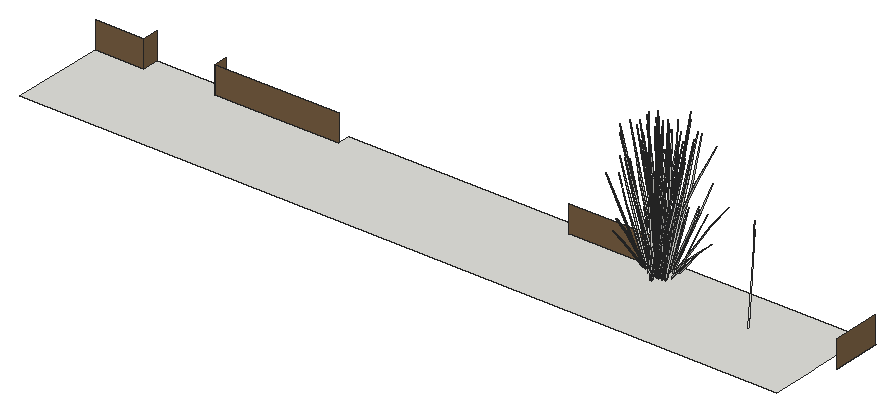
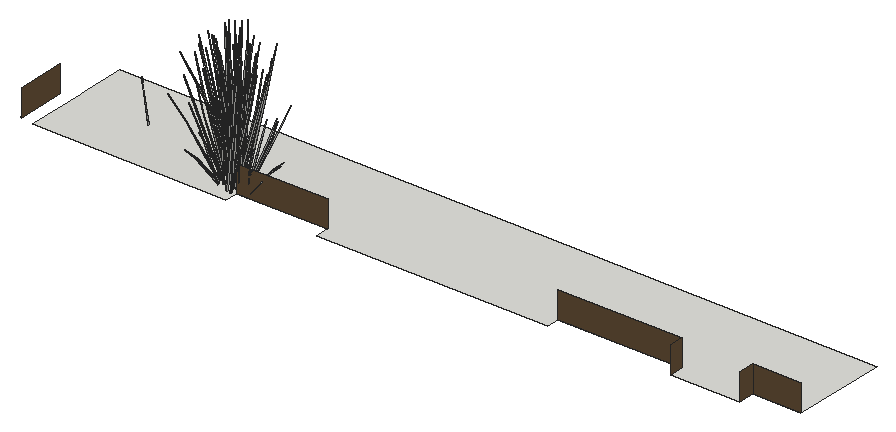
# SketchUp Ruby script. Lengths in inches.
U = 1.inch
M = Sketchup.active_model
def pt(a) = Geom::Point3d.new(a.map { |v| v * U })
def face(e, loops, mat)
  f = e.add_face(loops[0].map { |a| pt(a) })
  loops[1..].each { |l| e.add_face(l.map { |a| pt(a) }).erase! }
  f.material = f.back_material = mat if mat
  f
end
# faces: each face lists its corners as indices into pts; further lists are holes
def faces(e, pts, list, mat = nil) = list.each { |f| face(e, (f[0].is_a?(Array) ? f : [f]).map { |l| l.map { |i| pts[i] } }, mat) }
# xy, xz, yz: faces in a plane at the given z, y or x. An outline is a flat list of corners, or four numbers for a rectangle; further outlines are holes
def ring(l) = l.size == 4 ? [[l[0], l[1]], [l[2], l[1]], [l[2], l[3]], [l[0], l[3]]] : l.each_slice(2).to_a
def flat(e, list, mat, &to3) = list.each { |f| face(e, (f[0].is_a?(Array) ? f : [f]).map { |l| ring(l).map { |u, v| to3.(u, v) } }, mat) }
def xy(e, z, list, mat = nil) = flat(e, list, mat) { |x, y| [x, y, z] }
def xz(e, y, list, mat = nil) = flat(e, list, mat) { |x, z| [x, y, z] }
def yz(e, x, list, mat = nil) = flat(e, list, mat) { |y, z| [x, y, z] }
def lines(e, pts, list) = list.each { |a, b| e.add_line(pt(pts[a]), pt(pts[b])) }
# prism: a flat outline (further loops are holes) pulled along v
def prism(e, loops, v, mat = nil)
  f = face(e, loops, mat); d = Geom::Vector3d.new(v.map { |x| x * U })
  f.pushpull(f.normal.samedirection?(d) ? d.length : -d.length)
end
def box(e, o, s, mat = nil) = prism(e, [[o, [o[0] + s[0], o[1], o[2]], [o[0] + s[0], o[1] + s[1], o[2]], [o[0], o[1] + s[1], o[2]]]], [0, 0, s[2]], mat)
def at(x, y, z, deg = 0) = Geom::Transformation.translation(pt([x, y, z])) * Geom::Transformation.rotation(ORIGIN, Z_AXIS, deg.degrees)
def axes(o, x, y, z) = Geom::Transformation.new([*x, 0, *y, 0, *z, 0, *pt(o).to_a, 1])
def part(name) = M.definitions.add(name)
# library, detail: a bought-in or finely detailed component or shape, given as its bounding box
def library(name, o, s) = part(name).tap { |d| box(d.entities, o, s) }
def detail(e, o, s) = box(e.add_group.entities, o, s)
def put(e, d, t, mat = nil) = e.add_instance(d, t).tap { |i| i.material = mat if mat }
def group(e, t, mat = nil) = e.add_group.tap { |g| g.transformation = t; g.material = mat if mat }.entities
root = M.entities
M.materials.add("LightPink_Translucent").color = [144, 107, 117]
M.materials["LightPink_Translucent"].alpha = 0.75
M.materials.add("Soil_03_1K").color = [122, 96, 67]
c1 = part("blade")
p = [[2.15,0.21,22],[0,0.17,0],[0.09,0.45,0],[2.18,0.31,22],[2.29,0.31,22],[0.38,0.45,0],
  [2.48,0.24,33],[2.49,0.24,33],[2.48,0.22,33]]
faces(c1.entities,p,[[0,1,2,3],[4,5,2,3],[6,3,4,7],[8,0,3,6]])
c2 = part("blade with seeds\#1")
put(c2.entities,c1,at(0,0,0))
c3 = part("seeds")
p = [[0.3,-0.1,1.38],[-0.01,-0.03,1.59],[-0.01,-0.03,0.03],[0.14,-0.07,-0.07],[0.29,-0.03,3],[0.15,0.01,3.11]]
faces(c3.entities,p,[[0,1,2,3],[1,0,4,5]],"LightPink_Translucent")
c4 = part("blade with seeds")
put(c4.entities,c1,at(0,0,0))
put(c4.entities,c3,axes([2.4,0.25,30.99],[1.5799,-0.05474,1.17369],[-0.12525,1.92788,0.29478],[-0.07173,-0.02425,1.56792]))
xy(root,0,[[312.48,54.75,595.39,54.75,595.39,71.87,595,71.87,595,95.87,522.75,95.87,522.75,90.87,488.75,90.87,488.75,95.87,402.48,95.87,402.48,90.87,356.48,90.87,356.48,95.87,330.48,95.87,330.48,89.87,312.48,89.87],[600,76.87,600.39,94.87]])
xz(root,89.87,[[312.48,0,330.48,10]],"Soil_03_1K")
xz(root,90.87,[[356.48,0,402.48,10],[488.75,0,522.75,10]],"Soil_03_1K")
yz(root,330.48,[[89.87,0,95.87,10]],"Soil_03_1K")
yz(root,356.48,[[90.87,0,95.87,10]],"Soil_03_1K")
yz(root,600,[[76.87,0,94.87,10]],"Soil_03_1K")
put(root,c2,axes([524.77,85.99,1.1],[0.46619,-1.302,-0.26229],[0.98396,0.62692,-0.45076],[0.24158,-0.04092,1.43974]))
put(root,c2,axes([521.56,85.22,2.92],[-0.65648,0.82762,-0.46065],[-0.57493,-0.87428,-0.35681],[-0.33354,-0.12593,0.88141]))
put(root,c2,axes([521.42,88.76,0.52],[0.24175,-1.0786,-0.27926],[0.85134,0.27158,0.27926],[-0.09817,-0.21744,1.25283]))
put(root,c2,axes([523.69,87.3125,1.15],[-0.82007,0.69452,0.40331],[-0.57748,-1.05199,-0.1941],[0.10147,-0.22475,1.29492]))
put(root,c2,axes([524.71,85.62,1.05],[-0.28493,-1.07717,0.13053],[0.81364,-0.37722,-0.37274],[0.17907,0,1.14258]))
put(root,c2,axes([523.89,88.58,1.1],[-1.11485,0.13472,-0.26229],[-0.06741,-1.40314,-0.45076],[-0.1485,-0.24708,1.43974]))
put(root,c2,axes([525.88,83.16,0.52],[0.60959,0.80703,-0.27926],[-0.60959,0.80703,0.27926],[0.19635,0,1.25283]))
put(root,c2,axes([524.81,86.07,0.68],[0,-1.29348,0],[1.0115,0,0],[0,0,1.60831]))
put(root,c2,axes([525.77,85.47,0.58],[0.89455,-0.42392,-0.62393],[0.32217,1.22114,-0.16376],[0.30292,-0.04686,1.37722]))
put(root,c2,axes([524.29,86.49,0.84],[-0.20585,1.46124,0.44352],[-1.16261,-0.29738,0.17404],[0.11226,-0.21355,1.53985]))
put(root,c4,axes([566.17,77.21,1.78],[0.38672,-0.16338,1.43002],[0.95481,0.49262,-0.30754],[-0.28419,0.42626,0.61141]))
put(root,c2,axes([524.51,86.11,1.15],[-0.88038,-0.56093,0.40331],[0.4237,-1.16553,-0.1941],[0.20294,0,1.29492]))
put(root,c2,axes([528.72,88.26,2.92],[0.24493,-1.13649,-0.46065],[0.83975,0.38955,-0.35681],[0.33809,-0.10421,0.88141]))
put(root,c2,axes([527.5625,86.6,0.68],[0.43865,-1.16553,0],[0.91144,0.56093,0],[0,0,1.57718]))
put(root,c2,axes([525.24,86.1,0.69],[0.63109,-0.80703,0],[0.63109,0.80703,0],[0,0,1.52591]))
put(root,c2,axes([525.72,82.86,0.68],[-0.00781,1.44494,-0.04486],[-1.09198,0,0.45022],[0.24858,0.04541,1.42752]))
put(root,c2,axes([523.84,87.74,0.82],[0.88667,0.95859,0.41247],[-0.7827,1.13884,0.16186],[-0.08849,-0.2311,1.43206]))
put(root,c2,axes([522.4375,85.7,0.93],[0.25932,1.24233,0.15904],[-0.96507,0.30677,0.3163],[0.14061,-0.1108,1.44604]))
put(root,c2,axes([518.82,86.97,1.1875],[0.56973,-0.14831,1.03545],[-0.31555,0.82274,0.76078],[-0.29172,-0.08853,0.22807]))
put(root,c2,axes([521.1875,90,0.83],[-0.97904,0.72283,0],[-0.54599,-1.20931,-0.46523],[-0.12435,-0.27543,1.47583]))
put(root,c2,axes([528.57,88.67,3.1875],[0.79444,-0.5518,-0.64046],[0.44274,1.13586,0.07729],[0.38385,-0.12903,0.906]))
put(root,c2,axes([524.97,83.91,0.93],[-0.71168,0.90835,0.15904],[-0.69029,-0.91538,0.3163],[0.14534,0.10032,1.44604]))
put(root,c2,axes([527.19,87.02,0.76],[1.12244,-0.50265,-0.0542],[0.39331,1.43622,0],[0.0392,-0.01755,1.55211]))
put(root,c2,axes([524.56,87.05,0.68],[-1.1305,0,0],[0,-1.44565,0],[0,0,1.61777]))
put(root,c2,axes([524.1,88.81,1.15],[0.06031,1.25545,0.40331],[-1.00118,0.11354,-0.1941],[-0.10147,-0.22475,1.29492]))
put(root,c2,axes([522.38,89.4,0.93],[0.971,0.33398,0.15904],[-0.27478,1.22215,0.3163],[-0.00473,-0.21112,1.44604]))
put(root,c2,axes([525.01,86.32,0.76],[1.12994,0,-0.05082],[0,1.44565,0],[0.03551,0,1.61697]))
put(root,c2,axes([524.76,88.39,0.89],[0.47355,-1.30265,0.21694],[0.98396,0.62692,0.45076],[-0.22682,0,1.44726]))
put(root,c2,axes([525.5,86.13,0.6875],[0.88038,0.56093,-0.40331],[-0.4237,1.16553,0.1941],[0.20294,0,1.29492]))
put(root,c2,axes([527.17,87.65,0.68],[-0.84234,0.37722,0],[-0.29498,-1.07717,0],[0,0,1.39163]))
put(root,c2,axes([528.94,89.02,0.04],[-0.05317,-0.18711,1.5897],[0.29263,-1.12549,-0.24285],[0.32981,-0.03291,0.27078]))
put(root,c2,axes([520.41,87.16,2.78],[-0.75135,-0.34854,-0.31925],[0.21915,-1.01686,0.41216],[-0.30251,0.09324,0.78863]))
put(root,c2,axes([529.24,88.77,2.78],[0.75135,0.34854,-0.31925],[-0.21915,1.01686,0.41216],[0.30251,-0.09324,0.78863]))
put(root,c2,axes([527.97,85.48,0.93],[-0.48852,-1.08202,0.44759],[0.87598,-0.64674,0],[0.11126,0.24644,1.41987]))
put(root,c2,axes([524.33,89.09,0.6875],[-0.88038,-0.56093,-0.40331],[0.4237,-1.16553,0.1941],[-0.20294,0,1.29492]))
put(root,c2,axes([525.43,86.6875,0.77],[-0.84094,1.07538,-0.05527],[-0.84146,-1.07603,0],[-0.02937,0.03755,1.58274]))
put(root,c2,axes([528.03,86.1,0.8],[0.31757,-1.44738,0.27726],[1.13512,0.3621,-0.32897],[0.14207,0.23956,1.48641]))
put(root,c2,axes([524.47,88.86,0.82],[1.09253,-0.50265,0.41247],[0.37991,1.43622,0.16186],[-0.20075,-0.01755,1.43206]))
put(root,c2,axes([519.32,88.21,0.04],[0.0352,0.19392,1.5897],[-0.39624,1.07238,-0.24285],[-0.33051,-0.01799,0.27078]))
put(root,c2,axes([527.45,85.82,0.93],[-0.971,-0.33398,0.15904],[0.27478,-1.22215,0.3163],[0.00473,0.21112,1.44604]))
put(root,c2,axes([525.73,86.41,1.15],[-0.06031,-1.25545,0.40331],[1.00118,-0.11354,-0.1941],[0.10147,0.22475,1.29492]))
put(root,c2,axes([526.16,86.38,1.05],[0.58702,-0.85413,0.13053],[0.66228,0.71246,-0.37274],[0.08953,0.19831,1.14258]))
put(root,c2,axes([527.55,87.92,0.68],[-0.43865,1.16553,0],[-0.91144,-0.56093,0],[0,0,1.46678]))
put(root,c2,axes([528.64,85.22,0.83],[0.97904,-0.72283,0],[0.54599,1.20931,-0.46523],[0.12435,0.27543,1.47583]))
put(root,c2,axes([527.39,89.52,0.93],[-0.25932,-1.24233,0.15904],[0.96507,-0.30677,0.3163],[-0.14061,0.1108,1.44604]))
put(root,c2,axes([521.08,87.26,3.1875],[-0.79444,0.5518,-0.64046],[-0.44274,-1.13586,0.07729],[-0.38385,0.12903,0.906]))
put(root,c2,axes([525.33,89.11,1.15],[0.88038,0.56093,0.40331],[-0.4237,1.16553,-0.1941],[-0.20294,0,1.29492]))
put(root,c2,axes([520.01,88.41,0.61],[0.56051,0.79893,-0.03509],[-0.61388,0.73204,-0.15911],[-0.17394,0.05154,0.52479]))
put(root,c2,axes([525.54,88.73,0.82],[0.20585,-1.46124,0.41247],[1.16261,0.29738,0.16186],[-0.11226,0.21355,1.43206]))
put(root,c2,axes([520.92,87.67,2.92],[-0.24493,1.13649,-0.46065],[-0.83975,-0.38955,-0.35681],[-0.33809,0.10421,0.88141]))
put(root,c2,axes([523.95,92.06,0.52],[-0.60959,-0.80703,-0.27926],[0.60959,-0.80703,0.27926],[-0.19635,0,1.25283]))
put(root,c2,axes([524.07,89.8125,0.59],[-1.0019,0.47479,-0.62955],[-0.36083,-1.36768,-0.16523],[-0.33927,0.05248,1.38963]))
put(root,c2,axes([525.94,86.64,1.1],[1.11485,-0.13472,-0.26229],[0.06741,1.40314,-0.45076],[0.1485,0.24708,1.43974]))
put(root,c2,axes([524.77,85.84,1.26],[-0.91991,0.03158,1.27354],[0.23846,-1.42935,0.53923],[0.50337,0.33806,1.20213]))
put(root,c2,axes([528.41,86.46,0.52],[-0.24175,1.0786,-0.27926],[-0.85134,-0.27158,0.27926],[0.09817,0.21744,1.25283]))
put(root,c2,axes([529.07,91.61,1.24],[-0.17302,-1.05027,0.05866],[0.69705,-0.24145,-0.77802],[0.35285,0.06658,0.69739]))
put(root,c2,axes([525.06,89.23,1.1],[-0.46619,1.302,-0.26229],[-0.98396,-0.62692,-0.45076],[-0.24158,0.04092,1.43974]))
put(root,c2,axes([528.53,86.13,0.67],[-0.98246,0.71382,-0.04636],[-0.54599,-1.20931,0.46523],[0.09354,0.298,1.4751]))
put(root,c2,axes([528.8,86.2,0.51],[0.48852,1.08202,-0.44759],[-0.87598,0.64674,0],[0.11126,0.24644,1.41987]))
put(root,c2,axes([528.09,90.71,3.21],[0.65648,-0.82762,-0.51132],[0.57493,0.87428,-0.39606],[0.33354,0.12593,0.97836]))
put(root,c2,axes([523.93,92.61,0.51],[-0.97703,0,-0.44759],[0,-1.29348,0],[-0.22253,0,1.41987]))
put(root,c2,axes([526.09,88.9,0.89],[-1.15773,-0.30643,-0.21121],[0.20181,-1.4529,0.4622],[-0.15988,0.25387,1.41028]))
put(root,c2,axes([526.37,88.37,1.05],[0.87196,0.22303,0.13053],[-0.15136,1.08968,-0.37274],[-0.08953,0.19831,1.14258]))
put(root,c2,axes([524.83,92.06,0.93],[0.97703,0,0.44759],[0,1.29348,0],[-0.22253,0,1.41987]))
put(root,c2,axes([529.0625,91.39,1.73],[-0.50438,-0.0254,1.3914],[0.26641,-1.14247,0.19228],[0.53755,0.09899,0.65702]))
put(root,c2,axes([526.21,87.52,0.6875],[0.06031,1.25545,-0.40331],[-1.00118,0.11354,0.1941],[0.10147,0.22475,1.29492]))
put(root,c2,axes([527.89,89.92,0.93],[0.48852,-1.08202,0.44759],[0.87598,0.64674,0],[-0.11126,0.24644,1.41987]))
put(root,c2,axes([526.38,86.95,0.92],[-0.78639,1.12892,-0.2271],[-0.88305,-0.94994,0.49699],[0.09199,0.304,1.51643]))
put(root,c2,axes([530.33,90.99,1.1875],[-0.58095,0.02992,1.03545],[0.41436,-0.74764,0.76078],[0.2769,0.14704,0.22807]))
put(root,c2,axes([525.62,89,0.6875],[-0.82007,0.69452,-0.40331],[-0.57748,-1.05199,0.1941],[-0.10147,0.22475,1.29492]))
